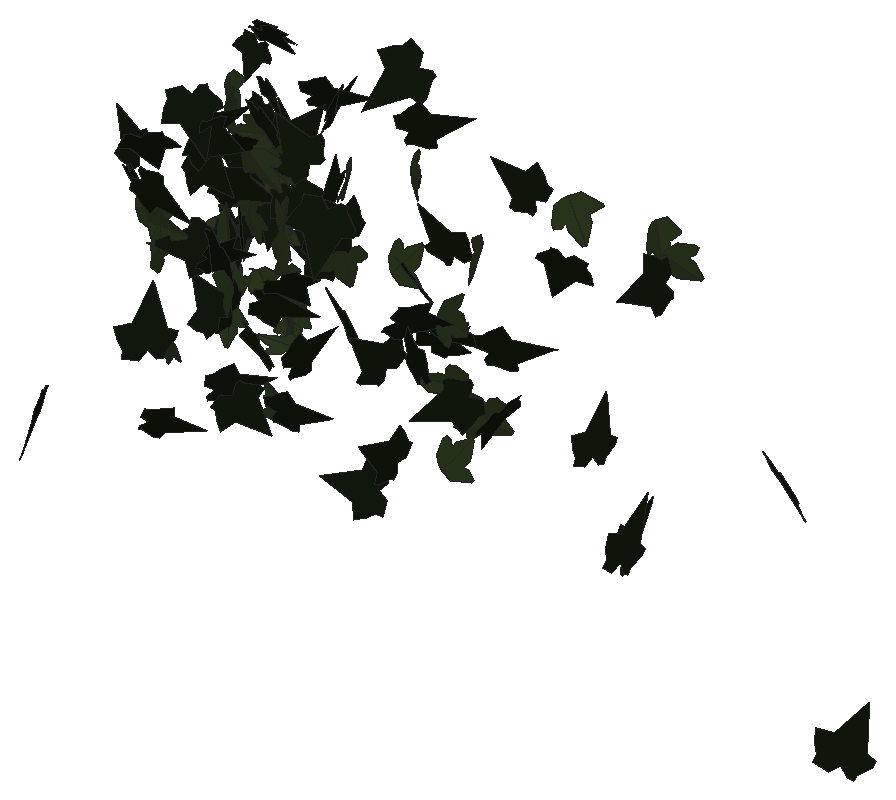
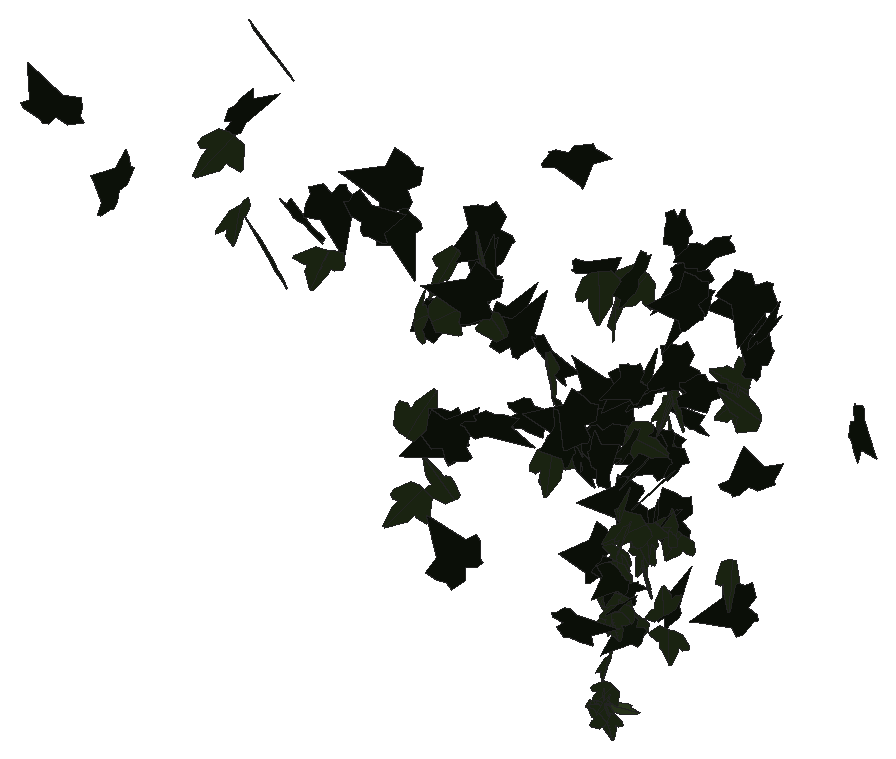
# SketchUp Ruby script. Lengths in inches.
U = 1.inch
M = Sketchup.active_model
def pt(a) = Geom::Point3d.new(a.map { |v| v * U })
def face(e, loops, mat)
  f = e.add_face(loops[0].map { |a| pt(a) })
  loops[1..].each { |l| e.add_face(l.map { |a| pt(a) }).erase! }
  f.material = f.back_material = mat if mat
  f
end
# faces: each face lists its corners as indices into pts; further lists are holes
def faces(e, pts, list, mat = nil) = list.each { |f| face(e, (f[0].is_a?(Array) ? f : [f]).map { |l| l.map { |i| pts[i] } }, mat) }
# xy, xz, yz: faces in a plane at the given z, y or x. An outline is a flat list of corners, or four numbers for a rectangle; further outlines are holes
def ring(l) = l.size == 4 ? [[l[0], l[1]], [l[2], l[1]], [l[2], l[3]], [l[0], l[3]]] : l.each_slice(2).to_a
def flat(e, list, mat, &to3) = list.each { |f| face(e, (f[0].is_a?(Array) ? f : [f]).map { |l| ring(l).map { |u, v| to3.(u, v) } }, mat) }
def xy(e, z, list, mat = nil) = flat(e, list, mat) { |x, y| [x, y, z] }
def xz(e, y, list, mat = nil) = flat(e, list, mat) { |x, z| [x, y, z] }
def yz(e, x, list, mat = nil) = flat(e, list, mat) { |y, z| [x, y, z] }
def lines(e, pts, list) = list.each { |a, b| e.add_line(pt(pts[a]), pt(pts[b])) }
# prism: a flat outline (further loops are holes) pulled along v
def prism(e, loops, v, mat = nil)
  f = face(e, loops, mat); d = Geom::Vector3d.new(v.map { |x| x * U })
  f.pushpull(f.normal.samedirection?(d) ? d.length : -d.length)
end
def box(e, o, s, mat = nil) = prism(e, [[o, [o[0] + s[0], o[1], o[2]], [o[0] + s[0], o[1] + s[1], o[2]], [o[0], o[1] + s[1], o[2]]]], [0, 0, s[2]], mat)
def at(x, y, z, deg = 0) = Geom::Transformation.translation(pt([x, y, z])) * Geom::Transformation.rotation(ORIGIN, Z_AXIS, deg.degrees)
def axes(o, x, y, z) = Geom::Transformation.new([*x, 0, *y, 0, *z, 0, *pt(o).to_a, 1])
def part(name) = M.definitions.add(name)
# library, detail: a bought-in or finely detailed component or shape, given as its bounding box
def library(name, o, s) = part(name).tap { |d| box(d.entities, o, s) }
def detail(e, o, s) = box(e.add_group.entities, o, s)
def put(e, d, t, mat = nil) = e.add_instance(d, t).tap { |i| i.material = mat if mat }
def group(e, t, mat = nil) = e.add_group.tap { |g| g.transformation = t; g.material = mat if mat }.entities
root = M.entities
M.materials.add("efeu1").color = [18, 25, 13]
M.materials.add("efeu2").color = [43, 57, 29]
c1 = part("ivyleaf_10")
p = [[0,0.5,-0.03],[-0.0625,2.02,-0.43],[-0.19,2.01,-0.46],[-0.54,1.05,-0.29],[-0.52,0.625,-0.18],[-0.83,0.76,-0.28],
  [-1.16,0.64,-0.33],[-1.15,0.33,-0.24],[-0.77,-0.39,0.02],[-0.3,-0.51,0.16],[0.04,-0.48,0.23],[-0.02,2.01,-0.4375],
  [-0.06,2.01,-0.43],[0.04,-0.49,0.23],[0.67,-0.49,0.14],[1.38,0.36,-0.2],[1.375,0.51,-0.24],[0.81,0.65,-0.19],
  [0.62,0.59,-0.15],[0.6,1.09,-0.28],[0.5,1.23,-0.31]]
faces(c1.entities,p,[[0,1,2,3,4,5,6,7,8,9,10],[11,12,0,13,14,15,16,17,18,19,20]],"efeu2")
c2 = part("ivyleaf_9")
p = [[1.54,2.16,1.25],[1.36,2.04,1.19],[-0.21,0.99,0.68],[-0.71,1.11,0.82],[-0.85,0.86,0.67],[-0.8,0.17,0.21],
  [-0.9,-0.01,0.1],[-0.67,-0.16,-0.02],[-0.08,-0.08,-0.05],[-0.03,-0.6,-0.4],[0.65,-0.88,-0.66],[0.83,-0.6,-0.49],
  [1.29,-0.42,-0.43],[1.8125,-0.07,-0.26],[1.21,0.44,0.15]]
faces(c2.entities,p,[[0,1,2,3,4,5,6,7,8,9,10,11,12,13,14]],"efeu1")
put(root,c1,axes([601.78,132.52,187.54],[0.96668,0.20887,0.10557],[0.08401,0.10907,-0.98503],[-0.21844,0.96629,0.08837]))
put(root,c1,axes([602,132.78,189.27],[0.29312,0.91321,-0.25171],[0.06644,0.24301,0.95905],[0.94494,-0.30037,0.01064]))
put(root,c2,axes([601.85,136.73,192.58],[-0.36731,-0.67676,-0.18819],[0.1313,0.14248,-0.76863],[0.69006,-0.38734,0.04608]))
put(root,c1,axes([602.37,126.25,188.94],[-0.96657,0.42032,0.4684],[-0.43428,0.17584,-1.05395],[-0.45549,-1.05959,0.01091]))
put(root,c1,axes([601.93,136.4,196.26],[-0.18294,0.76666,0.10713],[-0.00697,0.10844,-0.78797],[-0.77407,-0.18217,-0.01822]))
put(root,c2,axes([601.85,137.1,193.54],[0.53084,0.47884,0.32201],[0.09897,0.35551,-0.6918],[-0.56849,0.50901,0.18024]))
put(root,c2,axes([601.88,135.125,204.32],[-0.23141,-0.79533,0.20841],[0.02637,-0.22358,-0.82392],[0.82176,-0.21679,0.08513]))
put(root,c2,axes([601.68,136.07,199.76],[0.07935,-0.75562,0.34801],[0.11141,-0.33679,-0.75665],[0.82441,0.11824,0.06876]))
put(root,c1,axes([602.07,137.46,190.8],[0.67938,0.32894,-0.15258],[-0.18346,0.03232,-0.74722],[-0.31277,0.69556,0.10688]))
put(root,c2,axes([601.73,136.96,191.57],[0.20062,-0.68834,-0.34335],[0.00369,0.35569,-0.71093],[0.76922,0.17782,0.09296]))
put(root,c1,axes([601.99,138.48,184.63],[-0.00119,-0.56757,0.4258],[0.00069,0.4258,0.56757],[-0.70953,0.00136,-0.00016]))
put(root,c1,axes([602,132.65,202.91],[-0.23219,0.96823,0.01867],[-0.00056,0.01907,-0.99567],[-0.96841,-0.23216,-0.0039]))
put(root,c1,axes([602.08,137.27,191.2],[0.06234,0.72342,0.24404],[-0.105,0.25065,-0.7162],[-0.75622,0.02483,0.11956]))
put(root,c1,axes([602.19,136.99,193.85],[-0.78321,-0.11615,0.01117],[0.01427,-0.17059,-0.77313],[0.11581,-0.76449,0.17082]))
put(root,c1,axes([601.8125,136.875,191.23],[0.6962,0.17225,0.32875],[0.24238,0.31821,-0.68003],[-0.28106,0.70109,0.22788]))
put(root,c1,axes([602.08,134.45,192.52],[0.59558,-0.63739,0.07321],[0.04865,-0.05473,-0.87234],[0.63973,0.59756,-0.00182]))
put(root,c1,axes([602,136.96,191.72],[-0.62725,-0.38994,-0.28867],[0.2996,0.0598,-0.73177],[0.38161,-0.68789,0.10002]))
put(root,c1,axes([602.12,137.91,184.37],[0.71891,0.11344,-0.10595],[-0.11411,0.04596,-0.72512],[-0.10523,0.72522,0.06253]))
put(root,c1,axes([602.07,138.03,185.51],[-0.13167,0.69238,-0.08177],[0.00568,-0.08215,-0.70472],[-0.69717,-0.13143,0.0097]))
put(root,c1,axes([602.1,136.17,198.27],[-0.30964,0.74695,0.02492],[-0.00552,0.02469,-0.80857],[-0.74734,-0.30966,-0.00435]))
put(root,c1,axes([602.08,136.69,194.53],[0.67938,-0.38508,0.03991],[0.05019,0.00769,-0.78029],[0.38387,0.68051,0.0314]))
put(root,c1,axes([601.68,131.74,193.68],[0.82566,0.30023,0.54458],[0.51822,0.16817,-0.8784],[-0.34374,0.97468,-0.01619]))
put(root,c2,axes([601.8,133.18,198.04],[0.59442,-0.56889,-0.413],[-0.09858,0.46805,-0.78661],[0.69605,0.55212,0.24129]))
put(root,c2,axes([602.3,136.94,193.8125],[0.32528,0.71981,-0.02665],[-0.01486,-0.02253,-0.78989],[-0.72015,0.32559,0.00426]))
put(root,c1,axes([602.41,133.93,194.84],[-0.5064,-0.73834,0.06604],[-0.03721,-0.05455,-0.89531],[0.74035,-0.50777,0.00017]))
put(root,c1,axes([602.22,137.79,188.1],[-0.14105,0.7349,0.02508],[-0.03209,0.01936,-0.74779],[-0.73462,-0.14195,0.02785]))
put(root,c1,axes([602.98,136.37,184.1875],[-0.0119,0.91215,0.07957],[-0.88064,-0.03318,0.24871],[0.25064,-0.07329,0.87767]))
put(root,c2,axes([602.11,135.4375,189.23],[0.80816,0.32085,0.07328],[-0.08749,0.39675,-0.77225],[-0.31727,0.70787,0.39962]))
put(root,c1,axes([602.1,137.84,186.16],[-0.55055,-0.22208,-0.45068],[0.43421,0.12605,-0.59254],[0.25277,-0.70023,0.03627]))
put(root,c1,axes([602.1,136.87,194.89],[0.73948,0.07386,0.24658],[0.23873,0.08374,-0.741],[-0.09627,0.775,0.05657]))
put(root,c1,axes([602.19,137.97,185.61],[0.35517,-0.45589,0.46148],[0.30976,-0.34308,-0.57732],[0.56996,0.47055,0.02618]))
put(root,c2,axes([602.76,123.01,202.79],[-0.262,-0.95181,0.45422],[0.13394,0.43421,0.98713],[-1.0461,0.29398,0.01263]))
put(root,c1,axes([602.84,131.37,201.79],[-0.19462,0.26516,0.99656],[-0.55949,0.82477,-0.32872],[-0.86627,-0.59226,-0.01159]))
put(root,c1,axes([602.53,133.89,193.67],[-0.87465,0.18745,-0.06691],[0.06487,-0.01663,-0.89451],[-0.18816,-0.87705,0.00266]))
put(root,c2,axes([601.99,135.22,205.51],[0.80528,0.05569,0.29584],[0.28829,0.1006,-0.80366],[-0.08668,0.85198,0.07556]))
put(root,c1,axes([602.52,138.18,185.15],[0.70795,0.09119,-0.06828],[-0.07027,0.01132,-0.71351],[-0.08966,0.71114,0.02012]))
put(root,c2,axes([602.11,135.7,201.51],[0.51261,-0.65051,0.08874],[0.0407,-0.08088,-0.82802],[0.65528,0.51391,-0.01799]))
put(root,c1,axes([601.88,132.07,194.17],[0.04006,-0.13965,0.93591],[0.93644,-0.12885,-0.0593],[0.13607,0.92786,0.13263]))
put(root,c2,axes([602.6,131.84,188.36],[0.06127,0.09611,1.11467],[-0.51255,-0.98989,0.11352],[0.99449,-0.5161,-0.01016]))
put(root,c2,axes([602.4,135.19,205.38],[0.82916,0.26779,0.07465],[0.07284,0.01735,-0.87131],[-0.26829,0.83233,-0.00585]))
put(root,c1,axes([602.14,135.06,195.7],[0.47201,0.35225,1.01171],[0.7455,0.68594,-0.58664],[-0.76933,0.88082,0.05225]))
put(root,c1,axes([602.51,134.71,189.3],[0.62688,0.30394,0.50272],[0.42759,0.26806,-0.69527],[-0.40283,0.75753,0.04432]))
put(root,c2,axes([602.49,132.49,199.26],[0.86462,0.18398,0.3408],[0.32401,0.11309,-0.88305],[-0.21216,0.92245,0.04029]))
put(root,c1,axes([603.99,132.94,200.09],[0.23356,0.08458,-1.10888],[-1.10338,0.15928,-0.22025],[0.13904,1.12196,0.11487]))
put(root,c2,axes([602.81,131.98,194.3125],[0.14145,-1.01284,0.08061],[0.0047,-0.08074,-1.02265],[1.01603,0.14138,-0.00649]))
put(root,c1,axes([602.34,124.34,198.45],[0.33059,-0.1268,-1.21528],[1.17894,-0.29772,0.35177],[-0.32107,-1.22375,0.04034]))
put(root,c2,axes([603.75,131.29,194.56],[0.31825,-0.03539,-1.05977],[-1.00598,0.33971,-0.31344],[0.33521,1.05309,0.0655]))
put(root,c2,axes([604.71,138.48,189.95],[-0.73426,-0.50863,-0.84883],[-0.69806,-0.48293,0.89322],[-0.70137,1.01313,-0.00038]))
put(root,c2,axes([603.08,122.54,200.87],[0.27508,-0.4292,1.06823],[0.68229,-0.82385,-0.5067],[0.92726,0.73352,0.05594]))
put(root,c2,axes([603.375,123.49,184.91],[0.81953,0.28047,0.73328],[0.69822,0.22428,-0.86613],[-0.35896,1.07659,-0.01059]))
put(root,c2,axes([604.33,121.52,204.91],[0.81994,0.85897,-0.30443],[-0.23224,-0.19904,-1.18712],[-0.88123,0.85169,0.0296]))
put(root,c2,axes([604.36,112.06,191.79],[-0.61981,0.41507,-1.02408],[0.84997,-0.57121,-0.74595],[-0.70609,-1.05196,0.00099]))
put(root,c2,axes([603.875,129.93,198.27],[0.12202,0.11892,-1.14603],[0.53579,1.0144,0.16231],[1.02003,-0.54706,0.05184]))
put(root,c2,axes([605.29,134.79,198.44],[0.21935,-0.38978,1.09812],[-0.53942,0.9565,0.44726],[-1.03287,-0.58232,-0.00038]))
put(root,c2,axes([604.96,121.19,191.46],[-0.87518,-0.54852,0.80717],[0.67672,0.44009,1.03281],[-0.70316,1.10624,-0.01065]))
put(root,c1,axes([604.96,122.03,197.51],[-0.00091,-0.07634,-1.22885],[0.1881,1.21441,-0.07558],[1.21676,-0.18779,0.01076]))
put(root,c1,axes([604.48,122.5,198.77],[-0.14387,-0.1178,1.17235],[1.16205,0.18101,0.16079],[-0.19473,1.16719,0.09339]))
put(root,c1,axes([605.3,127.84,197.2],[0.58332,-0.32814,0.96519],[0.85246,-0.45286,-0.66915],[0.55909,1.03285,0.01325]))
put(root,c2,axes([606.37,136.24,200.66],[0.15861,0.38807,1.13311],[0.27592,1.10042,-0.4155],[-1.16551,0.31332,0.05584]))
put(root,c2,axes([605.48,136.05,201.8],[0.65317,-0.08747,1.00708],[1.01084,0.04732,-0.6515],[0.00775,1.19941,0.09914]))
put(root,c2,axes([605.51,120.22,203],[0.14372,0.09682,-1.25133],[1.09428,0.60712,0.17265],[0.61461,-1.10358,-0.0148]))
put(root,c2,axes([606.11,124.66,204.61],[0.28144,0.27325,1.10202],[0.83964,0.71418,-0.39151],[-0.76428,0.88522,-0.0243]))
put(root,c2,axes([607.3125,123.76,197.93],[-0.33577,-0.64961,-0.93352],[-0.34002,-0.87149,0.72875],[-1.08528,0.47402,0.0605]))
put(root,c2,axes([606.56,123.32,207.66],[-0.14356,-1.13895,-0.59227],[0.08247,0.58655,-1.14794],[1.28109,-0.16539,0.00753]))
put(root,c2,axes([607.17,123.38,203.96],[0.36163,-0.65673,-1.02545],[-0.43434,0.92979,-0.74864],[1.13762,0.56375,0.04015]))
put(root,c2,axes([607.48,123.08,205.45],[0.1228,-0.0497,-1.1794],[-0.27448,1.15206,-0.07713],[1.14809,0.28075,0.10771]))
put(root,c2,axes([607.25,131.67,201.0625],[-0.5473,0.13761,0.99211],[0.96183,-0.24325,0.56434],[0.27947,1.10664,0.00068]))
put(root,c2,axes([607.8125,131.22,198.4],[-0.10722,-0.83999,-0.77111],[0.06563,0.76868,-0.84647],[1.13837,-0.12344,-0.02383]))
put(root,c2,axes([609.14,140.85,202.77],[-1.18789,-0.57412,0.37967],[-0.33746,-0.17424,-1.31932],[0.5999,-1.23486,0.00964]))
put(root,c2,axes([607.875,128.16,192.41],[0.34021,0.381,-1.06977],[0.67947,0.82649,0.51044],[0.90988,-0.75965,0.01881]))
put(root,c2,axes([609.73,131.43,196.02],[-0.35087,0.42429,1.19477],[-0.83946,0.85129,-0.54884],[-0.95016,-0.90879,0.04369]))
put(root,c2,axes([609.57,121.91,194.83],[-1.01812,-0.10373,-0.49978],[-0.49703,-0.05239,1.02339],[-0.1162,1.13296,0.00156]))
put(root,c1,axes([609.3,128.53,185.22],[-1.0075,0.02707,-0.55302],[-0.55341,-0.01347,1.00756],[0.01724,1.14922,0.02484]))
put(root,c2,axes([608.32,123.46,188.88],[0.551,0.29744,1.04548],[0.93603,0.46604,-0.62591],[-0.55259,1.08602,-0.01774]))
put(root,c2,axes([608.85,122.0625,198.35],[0.59218,0.6415,0.72569],[0.50042,0.52561,-0.873],[-0.82928,0.77526,-0.0086]))
put(root,c1,axes([609.79,122.45,196.63],[0.86314,-0.66882,-0.56296],[-0.42473,0.37065,-1.09155],[0.7641,0.96154,0.02919]))
put(root,c2,axes([610.25,131.4,198.47],[-0.88004,0.56746,-0.81112],[-0.70887,0.39629,1.04635],[0.69096,1.12931,0.04039]))
put(root,c2,axes([609.05,126.5,206.01],[0.81943,-0.9613,0.3054],[0.19996,-0.23086,-1.26315],[0.98862,0.84347,0.00234]))
put(root,c2,axes([609.62,128.97,188.51],[0.11196,0.17922,1.19397],[0.76559,0.91665,-0.20938],[-0.93357,0.77321,-0.02852]))
put(root,c1,axes([610.48,124.4,204.5],[-1.01275,0.0091,-0.62295],[0.62297,0.00121,-1.01278],[-0.00712,-1.189,-0.0058]))
put(root,c1,axes([611.625,131.17,195.4],[-0.63754,-0.94943,-0.20202],[0.1255,0.15905,-1.14352],[0.96254,-0.64959,0.01529]))
put(root,c1,axes([611.84,126.57,204.83],[-0.73153,-0.96042,0.00524],[-0.00175,-0.00525,-1.20729],[0.96044,-0.73153,0.00179]))
put(root,c2,axes([611.74,125.16,196.44],[0.83685,0.85483,-0.00621],[-0.00902,0.00015,-1.19625],[-0.85481,0.83687,0.00655]))
put(root,c1,axes([612.14,130.74,201.23],[0.46187,-0.99398,-0.39492],[-0.1642,0.35918,-1.09604],[1.05688,0.49018,0.0023]))
put(root,c2,axes([613.16,125.73,204.64],[-1.04121,-0.48177,-0.21139],[-0.19125,-0.09006,1.14727],[-0.49012,1.05863,0.0014]))
put(root,c1,axes([613.09,123.39,201.23],[-0.02269,0.26617,-1.21831],[-0.36841,1.1627,0.26088],[1.19139,0.36461,0.05747]))
put(root,c2,axes([612.42,119.91,191.28],[0.05711,-0.50346,-1.05805],[-0.0162,1.05886,-0.50472],[1.17161,0.03918,0.04459]))
put(root,c2,axes([613.09,121.4,194.29],[0.83329,-0.79717,-0.25299],[0.18517,-0.17242,1.15319],[-0.8156,-0.85361,0.00333]))
put(root,c2,axes([614.58,127.875,199.38],[-0.31428,0.32401,1.14201],[-0.80327,0.81177,-0.45137],[-0.87404,-0.86255,0.00419]))
put(root,c2,axes([614.24,116.18,203.53],[0.5615,0.09489,-1.07433],[-1.07038,-0.09938,-0.56822],[-0.13215,1.20813,0.03764]))
put(root,c1,axes([613.97,122.54,200.14],[-0.49655,0.75485,0.81094],[0.45917,-0.66853,0.90345],[1.00826,0.6762,-0.01206]))
put(root,c2,axes([614.57,128.29,192.4],[0.4013,-1.0213,0.56979],[-0.21303,0.52849,1.09731],[-1.14993,-0.45432,-0.00443]))
put(root,c2,axes([614.87,135.28,188.86],[1.04758,0.60752,-0.22983],[0.19529,0.12137,1.21098],[0.61949,-1.06561,0.0069]))
put(root,c2,axes([614.78,121.08,190.625],[0.58221,-0.08392,1.00036],[0.98708,-0.16281,-0.58814],[0.18288,1.14594,-0.0103]))
put(root,c2,axes([616.74,134.7,195.85],[0.51985,-0.27528,1.09128],[-0.96986,0.50031,0.58821],[-0.57101,-1.10038,-0.00556]))
put(root,c2,axes([615.77,132.21,204.78],[0.41369,0.10407,1.21451],[1.20021,0.18934,-0.42505],[-0.21301,1.26899,-0.03618]))
put(root,c1,axes([618.72,128.71,204.66],[0.18768,-0.2549,-1.14409],[0.63836,-0.94953,0.31628],[-0.98307,-0.66525,-0.01305]))
put(root,c1,axes([619.18,126.76,199.28],[0.92194,-0.24677,-0.78772],[0.76446,-0.19032,0.95434],[-0.31146,-1.19761,0.01065]))
put(root,c2,axes([619.47,130.33,193.77],[1.05901,0.1704,0.5293],[0.5222,0.08642,-1.07263],[-0.19104,1.18077,0.00212]))
put(root,c2,axes([620.35,118.59,206.91],[-0.75984,-1.0919,-0.33191],[0.1823,0.2775,-1.33023],[1.12657,-0.78135,-0.00861]))
put(root,c2,axes([621.66,122.29,195.47],[0.24514,0.29945,1.19139],[-0.96127,-0.70966,0.37616],[0.76487,-0.98786,0.09092]))
put(root,c2,axes([621.7,125.05,199.95],[1.05238,-0.65689,-0.06147],[0.0793,0.01106,1.2395],[-0.65497,-1.05412,0.05131]))
put(root,c2,axes([623.25,119.54,189.05],[-0.59194,-0.48871,-0.9175],[-0.65838,-0.64083,0.7661],[-0.80447,0.88405,0.04813]))
put(root,c1,axes([622.22,130.54,188.72],[-0.56397,-0.56407,-0.90508],[0.62026,0.65937,-0.79744],[0.86753,-0.83813,-0.01823]))
put(root,c1,axes([622.45,129.97,200.07],[0.1927,-0.31179,1.15088],[0.71041,-0.90628,-0.36448],[0.95763,0.73506,0.0388]))
put(root,c1,axes([622.67,127.04,187.35],[0.9456,-0.12598,-0.74227],[0.73552,-0.0999,0.95396],[-0.16078,-1.19798,-0.00149]))
put(root,c1,axes([624.9375,127.46,191.08],[-0.81838,-0.62266,-0.7283],[-0.56908,-0.45472,1.02823],[-0.7709,0.99669,0.01412]))
put(root,c2,axes([624.82,119.69,200.72],[0.80317,0.7267,0.76336],[0.57424,0.50305,-1.08309],[-0.88377,0.98729,-0.01001]))
put(root,c2,axes([626.125,119.93,197.77],[0.34157,-0.47745,1.19621],[-0.54891,1.06558,0.58205],[-1.16515,-0.64197,0.07647]))
put(root,c1,axes([625.71,122.9,199.89],[-0.14684,0.84859,0.92094],[-0.20657,0.89813,-0.86051],[-1.23513,-0.2511,0.03443]))
put(root,c2,axes([626.68,129.8,205.19],[-0.12747,0.05752,1.21771],[-1.04927,0.61812,-0.13903],[-0.62061,-1.05688,-0.01504]))
put(root,c2,axes([626.0625,117.78,192.74],[0.08362,0.08942,1.2258],[-0.78196,-0.94402,0.12221],[0.94822,-0.78638,-0.00732]))
put(root,c1,axes([626.53,122.73,195.79],[-0.30793,-0.25474,-1.15462],[-0.92712,-0.68848,0.39915],[-0.73383,0.97672,-0.01978]))
put(root,c2,axes([627.625,122.46,195.48],[-0.13997,-0.28727,-1.18433],[-0.13731,-1.18081,0.30264],[-1.21091,0.1671,0.10258]))
put(root,c1,axes([627.38,132.47,203.71],[0.76219,0.8917,0.39726],[0.26814,0.29338,-1.17299],[-0.93864,0.80789,-0.0125]))
put(root,c2,axes([631.28,126.91,203.94],[0.65606,0.56023,-0.89357],[-0.66733,-0.59441,-0.86261],[-0.8167,0.93572,-0.01297]))
put(root,c2,axes([633.17,118.57,198.08],[-0.32273,1.1635,-0.38276],[0.10281,-0.36869,-1.20743],[-1.22052,-0.33872,-0.0005]))
put(root,c2,axes([631.71,119.75,201.13],[0.57661,-0.0393,1.19422],[1.19469,0.04229,-0.57545],[-0.02102,1.32547,0.05377]))
put(root,c1,axes([633.9,132.4,204.375],[0.01285,1.26224,-0.10688],[-0.01057,-0.10677,-1.26227],[-1.26671,0.0137,0.00945]))
put(root,c1,axes([637.91,128.5,205.74],[-0.72282,-0.60275,-0.85395],[0.65753,0.54488,-0.94116],[0.81252,-0.97714,0.00195]))
put(root,c2,axes([638.74,120.29,196.61],[-1.12836,0.5835,0.09378],[0.08335,-0.04298,1.2703],[0.58508,1.13144,-0.00011]))
put(root,c2,axes([639.43,125.88,205.67],[-0.33077,-0.54169,1.10762],[-0.61204,-0.92339,-0.63436],[1.07035,-0.69541,-0.02045]))
put(root,c2,axes([642.41,118.42,191.79],[-0.7137,1.09514,0.52343],[0.25582,-0.45785,1.30676],[1.18654,0.75745,0.0331]))
put(root,c2,axes([650.1,108.72,198.63],[-1.03886,0.95051,0.26711],[0.1916,-0.18629,1.40806],[0.96856,1.05635,0.00796]))
put(root,c2,axes([649.14,124.49,197.04],[0.63505,-0.91114,0.82224],[0.48167,-0.66649,-1.11055],[1.12882,0.79698,0.0113]))
put(root,c2,axes([665.38,110,189.98],[-0.95601,0.13412,0.99079],[0.96355,-0.24232,0.96253],[0.26688,1.35532,0.07405]))
